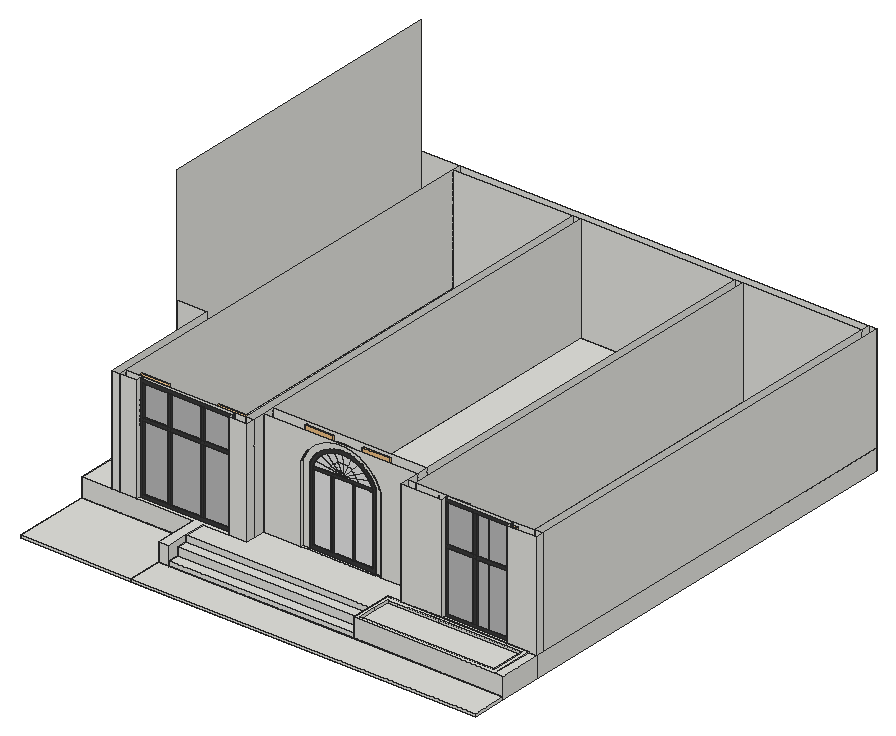
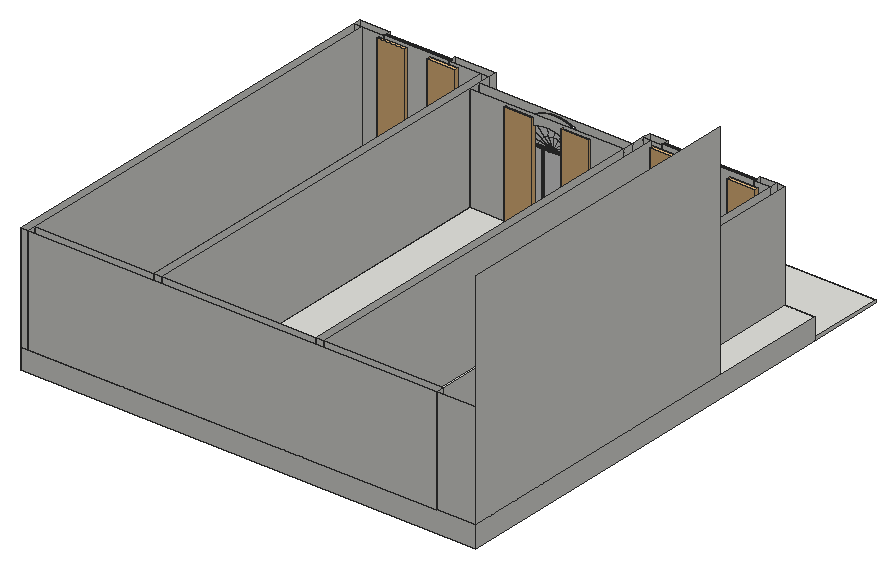
# SketchUp Ruby script. Lengths in inches.
U = 1.inch
M = Sketchup.active_model
def pt(a) = Geom::Point3d.new(a.map { |v| v * U })
def face(e, loops, mat)
  f = e.add_face(loops[0].map { |a| pt(a) })
  loops[1..].each { |l| e.add_face(l.map { |a| pt(a) }).erase! }
  f.material = f.back_material = mat if mat
  f
end
# faces: each face lists its corners as indices into pts; further lists are holes
def faces(e, pts, list, mat = nil) = list.each { |f| face(e, (f[0].is_a?(Array) ? f : [f]).map { |l| l.map { |i| pts[i] } }, mat) }
# xy, xz, yz: faces in a plane at the given z, y or x. An outline is a flat list of corners, or four numbers for a rectangle; further outlines are holes
def ring(l) = l.size == 4 ? [[l[0], l[1]], [l[2], l[1]], [l[2], l[3]], [l[0], l[3]]] : l.each_slice(2).to_a
def flat(e, list, mat, &to3) = list.each { |f| face(e, (f[0].is_a?(Array) ? f : [f]).map { |l| ring(l).map { |u, v| to3.(u, v) } }, mat) }
def xy(e, z, list, mat = nil) = flat(e, list, mat) { |x, y| [x, y, z] }
def xz(e, y, list, mat = nil) = flat(e, list, mat) { |x, z| [x, y, z] }
def yz(e, x, list, mat = nil) = flat(e, list, mat) { |y, z| [x, y, z] }
def lines(e, pts, list) = list.each { |a, b| e.add_line(pt(pts[a]), pt(pts[b])) }
# prism: a flat outline (further loops are holes) pulled along v
def prism(e, loops, v, mat = nil)
  f = face(e, loops, mat); d = Geom::Vector3d.new(v.map { |x| x * U })
  f.pushpull(f.normal.samedirection?(d) ? d.length : -d.length)
end
def box(e, o, s, mat = nil) = prism(e, [[o, [o[0] + s[0], o[1], o[2]], [o[0] + s[0], o[1] + s[1], o[2]], [o[0], o[1] + s[1], o[2]]]], [0, 0, s[2]], mat)
def at(x, y, z, deg = 0) = Geom::Transformation.translation(pt([x, y, z])) * Geom::Transformation.rotation(ORIGIN, Z_AXIS, deg.degrees)
def axes(o, x, y, z) = Geom::Transformation.new([*x, 0, *y, 0, *z, 0, *pt(o).to_a, 1])
def part(name) = M.definitions.add(name)
# library, detail: a bought-in or finely detailed component or shape, given as its bounding box
def library(name, o, s) = part(name).tap { |d| box(d.entities, o, s) }
def detail(e, o, s) = box(e.add_group.entities, o, s)
def put(e, d, t, mat = nil) = e.add_instance(d, t).tap { |i| i.material = mat if mat }
def group(e, t, mat = nil) = e.add_group.tap { |g| g.transformation = t; g.material = mat if mat }.entities
root = M.entities
M.materials.add("[Color M07]").color = [58, 58, 58]
M.materials.add("[Mirror 01]").color = [185, 185, 185]
M.materials.add("[Mirror 02]").color = [229, 229, 229]
c1 = library("Curtains 004",[-15.59,-2.26,0],[31.18,4.52,116.91])
xy(root,-24,[[2.97,0,128.4,86.25],[128.4,0,517.41,38.25],[128.4,38.25,128.4,86.25,2.97,86.25,2.97,566.25,517.41,566.25,517.41,86.25,140.65,86.25,140.65,38.25],[140.65,38.25,348.83,86.25],[348.83,38.25,517.41,86.25]])
xy(root,-20.66,[[2.97,0,128.4,86.25],[128.4,0,517.41,38.25]])
xy(root,-15.28,[[140.65,38.25,348.83,50.25]])
xy(root,-6.56,[[140.65,50.25,348.83,62.25]])
xy(root,-2.4375,[[353.04,42.45,504.2,82.05]])
xy(root,0,[[128.4,38.25,140.65,38.25,140.65,86.25,169.68,86.25,169.68,90.75,65.51,90.75,65.51,86.25,128.4,86.25],[508.41,38.25,517.41,86.25],[140.65,62.25,348.83,62.25,348.83,86.25,364.41,86.25,364.41,109.85,190.41,109.85,190.41,86.25,140.65,86.25],[2.97,86.25,37.41,220.92],[37.41,86.25,37.41,220.92,2.97,220.92,2.97,566.25,46.41,566.25,46.41,86.25],
  [46.41,86.25,65.51,95.25],[169.68,86.25,190.41,95.25],[364.41,86.25,409.78,95.25],[409.78,86.25,483.95,90.75],[483.95,86.25,508.41,95.25],
  [508.41,86.25,517.41,95.25],[46.41,95.25,181.41,557.25],[181.41,95.25,190.41,557.25],[364.41,95.25,373.41,557.25],[373.41,95.25,508.41,557.25],
  [508.41,95.25,517.41,566.25],[232.59,109.85,239.71,112.66],[239.71,109.85,314.84,112.66],[314.84,109.85,321.96,112.66],[239.71,113.47,314.84,122.61],
  [190.41,122.61,364.41,557.25],[46.41,557.25,508.41,566.25]])
xy(root,0,[[65.51,90.75,169.68,94.4375],[409.78,90.75,483.95,94.5625],[239.71,112.66,314.84,113.47]],"[Color M07]")
xy(root,0.875,[[[348.83,38.25,508.41,86.25],[353.04,42.45,504.2,82.05]]])
xy(root,3.13,[[412.91,90.75,441.92,92.125],[446.86,90.75,480.82,92.125]],"[Color M07]")
xy(root,3.65,[[69.16,90.75,96.8,92.5625],[100.57,90.75,134.3,92.5625],[137.83,90.75,166.03,92.5625]],"[Color M07]")
xy(root,3.99,[[263.76,112.66,266.13,113.47],[288.32,112.66,290.13,113.47]])
xy(root,3.99,[[243.71,112.66,263.76,113.47],[266.13,112.66,288.32,113.47],[290.13,112.66,310.84,113.47]],"[Color M07]")
xy(root,70.47,[[412.91,90.75,441.92,92.125],[446.86,90.75,480.82,92.125]],"[Color M07]")
xy(root,74.03,[[412.91,90.75,441.92,92.125],[446.86,90.75,480.82,92.125]],"[Color M07]")
xy(root,78.26,[[69.16,90.75,96.8,92.5625],[100.57,90.75,134.3,92.5625],[137.83,90.75,166.03,92.5625]],"[Color M07]")
xy(root,81.33,[[243.71,112.66,263.76,113.47],[266.13,112.66,288.32,113.47],[290.13,112.66,310.84,113.47]],"[Color M07]")
xy(root,81.69,[[69.16,90.75,96.8,92.5625],[100.57,90.75,134.3,92.5625],[137.83,90.75,166.03,92.5625]],"[Color M07]")
xz(root,0,[[2.97,-24,128.4,-20.66],[128.4,-24,517.41,-20.66]])
xz(root,38.25,[[128.4,-24,140.65,-20.66],[140.65,-24,348.83,-20.66],[348.83,-24,517.41,-20.66],[128.4,-20.66,140.65,0],[140.65,-20.66,348.83,-15.28],
  [348.83,-20.66,517.41,-20.66,517.41,0,508.41,0,508.41,0.875,348.83,0.875]])
xz(root,42.45,[[353.04,-2.4375,504.2,0.875]])
xz(root,50.25,[[140.65,-15.28,348.83,-6.56]])
xz(root,62.25,[[140.65,-6.56,348.83,0]])
xz(root,82.05,[[353.04,-2.4375,364.41,0.875],[364.41,-2.4375,409.78,0.875],[409.78,-2.4375,483.95,0.875],[483.95,-2.4375,504.2,0.875]])
xz(root,86.25,[[2.97,-24,128.4,-20.66],[348.83,-24,517.41,0],[2.97,-20.66,128.4,0],[37.41,0,46.41,120],[46.41,0,65.51,120],
  [169.68,0,190.41,120],[348.83,0,364.41,0.875],[364.41,0,409.78,0.875],[409.78,0,483.95,0.875],[483.95,0,508.41,0.875],
  [508.41,0,517.41,0,517.41,120,483.95,120,483.95,0.875,508.41,0.875],[364.41,0.875,409.78,120]])
xz(root,90.75,[[[65.51,0,169.68,120],[69.16,3.65,166.03,116.35]],[[409.78,0,483.95,120],[412.91,3.13,480.82,116.87]],[441.92,3.13,446.86,70.47],[96.8,3.65,100.57,78.26],[134.3,3.65,137.83,78.26],
  [412.91,70.47,441.92,74.03],[441.92,70.47,446.86,74.03],[446.86,70.47,480.82,74.03],[441.92,74.03,446.86,116.87],[69.16,78.26,96.8,81.69],
  [96.8,78.26,100.57,81.69],[100.57,78.26,134.3,81.69],[134.3,78.26,137.83,81.69],[137.83,78.26,166.03,81.69],[96.8,81.69,100.57,116.35],
  [134.3,81.69,137.83,116.35]],"[Color M07]")
xz(root,92.125,[[412.91,3.13,441.92,70.47],[446.86,3.13,480.82,70.47],[412.91,74.03,441.92,116.87],[446.86,74.03,480.82,116.87]],"[Mirror 01]")
xz(root,92.5625,[[69.16,3.65,96.8,78.26],[100.57,3.65,134.3,78.26],[137.83,3.65,166.03,78.26],[69.16,81.69,96.8,116.35],[100.57,81.69,134.3,116.35],
  [137.83,81.69,166.03,116.35]],"[Mirror 01]")
xz(root,94.4375,[[65.51,0,169.68,120]])
xz(root,94.5625,[[409.78,0,483.95,120]])
xz(root,95.25,[[46.41,0,65.51,120],[169.68,0,181.41,120],[181.41,0,190.41,120],[364.41,0,373.41,120],[373.41,0,409.78,120],
  [483.95,0,508.41,120],[508.41,0,517.41,120]])
xz(root,109.85,[[232.59,-7.12,321.96,0],[190.41,0,232.59,0,232.59,86.36,233.42,88.57,233.86,89.64,234.31,90.69,234.8,91.74,235.31,92.77,235.84,93.79,236.4,94.8,236.98,95.79,237.59,96.77,238.22,97.73,238.88,98.68,239.56,99.61,240.26,100.52,240.98,101.42,241.72,102.3,242.49,103.16,243.27,104,244.08,104.82,244.91,105.62,245.75,106.4,246.62,107.16,247.5,107.9,248.4,108.62,249.32,109.3125,250.25,109.99,251.2,110.64,252.17,111.26,253.15,111.86,254.15,112.44,255.16,112.99,256.18,113.52,257.21,114.03,258.26,114.5,259.32,114.96,260.39,115.38,261.47,115.78,262.56,116.15,263.66,116.5,264.76,116.82,265.88,117.11,267,117.38,268.125,117.62,269.26,117.83,270.39,118.01,271.53,118.16,272.68,118.29,273.83,118.39,274.97,118.46,276.125,118.5,277.28,118.51,278.43,118.5,279.58,118.46,280.73,118.39,281.875,118.29,283.02,118.16,284.16,118.01,285.3,117.83,286.43,117.62,287.55,117.38,288.67,117.11,289.79,116.82,290.89,116.5,291.99,116.15,293.08,115.78,294.16,115.38,295.23,114.96,296.29,114.5,297.34,114.03,298.37,113.52,299.4,112.99,300.41,112.44,301.4,111.86,302.38,111.26,303.35,110.64,304.3,109.99,305.23,109.3125,306.15,108.62,307.05,107.9,307.94,107.16,308.8,106.4,309.65,105.62,310.47,104.82,311.28,104,312.0625,103.16,312.83,102.3,313.57,101.42,314.3,100.52,315,99.61,315.67,98.68,316.33,97.73,316.96,96.77,317.57,95.79,318.15,94.8,318.71,93.79,319.24,92.77,319.75,91.74,320.24,90.69,320.7,89.64,321.13,88.57,321.96,86.36,321.96,0,364.41,0,364.41,120,190.41,120]])
xz(root,112.66,[[232.59,0,239.71,0,239.71,85.0625,240.06,85.98,240.42,86.88,240.8125,87.78,241.22,88.67,241.66,89.54,242.11,90.41,242.58,91.26,243.08,92.1,243.6,92.93,244.13,93.75,244.6875,94.56,245.26,95.35,245.86,96.12,246.47,96.88,247.1,97.63,247.75,98.36,248.42,99.07,249.1,99.77,249.8,100.45,250.52,101.11,251.25,101.76,252,102.38,252.77,102.99,253.55,103.58,254.34,104.15,255.15,104.71,255.97,105.24,256.8,105.75,257.65,106.24,258.5,106.71,259.37,107.16,260.25,107.58,261.14,107.99,262.04,108.37,262.94,108.73,263.86,109.07,264.79,109.39,265.72,109.68,266.66,109.95,267.6,110.2,268.55,110.43,269.51,110.63,270.47,110.81,271.43,110.96,272.4,111.09,273.375,111.2,274.35,111.28,275.32,111.34,276.3,111.38,277.28,111.39,278.25,111.38,279.23,111.34,280.2,111.28,281.18,111.2,282.15,111.09,283.12,110.96,284.08,110.81,285.04,110.63,286,110.43,286.95,110.2,287.9,109.95,288.83,109.68,289.77,109.39,290.69,109.07,291.61,108.73,292.51,108.37,293.41,107.99,294.3,107.58,295.18,107.16,296.05,106.71,296.91,106.24,297.75,105.75,298.58,105.24,299.4,104.71,300.21,104.15,301,103.58,301.78,102.99,302.55,102.38,303.3,101.76,304.03,101.11,304.75,100.45,305.45,99.77,306.13,99.07,306.8,98.36,307.45,97.63,308.08,96.88,308.7,96.12,309.29,95.35,309.87,94.56,310.42,93.75,310.96,92.93,311.47,92.1,311.97,91.26,312.44,90.41,312.9,89.54,313.33,88.67,313.74,87.78,314.13,86.88,314.49,85.98,314.84,85.0625,314.84,0,321.96,0,321.96,86.36,321.13,88.57,320.7,89.64,320.24,90.69,319.75,91.74,319.24,92.77,318.71,93.79,318.15,94.8,317.57,95.79,316.96,96.77,316.33,97.73,315.67,98.68,315,99.61,314.3,100.52,313.57,101.42,312.83,102.3,312.0625,103.16,311.28,104,310.47,104.82,309.65,105.62,308.8,106.4,307.94,107.16,307.05,107.9,306.15,108.62,305.23,109.3125,304.3,109.99,303.35,110.64,302.38,111.26,301.4,111.86,300.41,112.44,299.4,112.99,298.37,113.52,297.34,114.03,296.29,114.5,295.23,114.96,294.16,115.38,293.08,115.78,291.99,116.15,290.89,116.5,289.79,116.82,288.67,117.11,287.55,117.38,286.43,117.62,285.3,117.83,284.16,118.01,283.02,118.16,281.875,118.29,280.73,118.39,279.58,118.46,278.43,118.5,277.28,118.51,276.125,118.5,274.97,118.46,273.83,118.39,272.68,118.29,271.53,118.16,270.39,118.01,269.26,117.83,268.125,117.62,267,117.38,265.88,117.11,264.76,116.82,263.66,116.5,262.56,116.15,261.47,115.78,260.39,115.38,259.32,114.96,258.26,114.5,257.21,114.03,256.18,113.52,255.16,112.99,254.15,112.44,253.15,111.86,252.17,111.26,251.2,110.64,250.25,109.99,249.32,109.3125,248.4,108.62,247.5,107.9,246.62,107.16,245.75,106.4,244.91,105.62,244.08,104.82,243.27,104,242.49,103.16,241.72,102.3,240.98,101.42,240.26,100.52,239.56,99.61,238.88,98.68,238.22,97.73,237.59,96.77,236.98,95.79,236.4,94.8,235.84,93.79,235.31,92.77,234.8,91.74,234.31,90.69,233.86,89.64,233.42,88.57,232.59,86.36]])
xz(root,112.66,[[[239.71,0,314.84,0,314.84,85.0625,314.49,85.98,314.13,86.88,313.74,87.78,313.33,88.67,312.9,89.54,312.44,90.41,311.97,91.26,311.47,92.1,310.96,92.93,310.42,93.75,309.87,94.56,309.29,95.35,308.7,96.12,308.08,96.88,307.45,97.63,306.8,98.36,306.13,99.07,305.45,99.77,304.75,100.45,304.03,101.11,303.3,101.76,302.55,102.38,301.78,102.99,301,103.58,300.21,104.15,299.4,104.71,298.58,105.24,297.75,105.75,296.91,106.24,296.05,106.71,295.18,107.16,294.3,107.58,293.41,107.99,292.51,108.37,291.61,108.73,290.69,109.07,289.77,109.39,288.83,109.68,287.9,109.95,286.95,110.2,286,110.43,285.04,110.63,284.08,110.81,283.12,110.96,282.15,111.09,281.18,111.2,280.2,111.28,279.23,111.34,278.25,111.38,277.28,111.39,276.3,111.38,275.32,111.34,274.35,111.28,273.375,111.2,272.4,111.09,271.43,110.96,270.47,110.81,269.51,110.63,268.55,110.43,267.6,110.2,266.66,109.95,265.72,109.68,264.79,109.39,263.86,109.07,262.94,108.73,262.04,108.37,261.14,107.99,260.25,107.58,259.37,107.16,258.5,106.71,257.65,106.24,256.8,105.75,255.97,105.24,255.15,104.71,254.34,104.15,253.55,103.58,252.77,102.99,252,102.38,251.25,101.76,250.52,101.11,249.8,100.45,249.1,99.77,248.42,99.07,247.75,98.36,247.1,97.63,246.47,96.88,245.86,96.12,245.26,95.35,244.6875,94.56,244.13,93.75,243.6,92.93,243.08,92.1,242.58,91.26,242.11,90.41,241.66,89.54,241.22,88.67,240.8125,87.78,240.42,86.88,240.06,85.98,239.71,85.0625],[243.71,3.99,243.71,84.33,243.78,84.52,244.11,85.34,244.46,86.14,244.83,86.94,245.22,87.73,245.625,88.51,246.05,89.28,246.5,90.04,246.96,90.78,247.44,91.52,247.94,92.24,248.46,92.95,249,93.65,249.55,94.34,250.12,95.01,250.7,95.67,251.3,96.31,251.92,96.9375,252.55,97.55,253.2,98.15,253.86,98.73,254.53,99.29,255.22,99.84,255.92,100.37,256.63,100.88,257.36,101.38,258.1,101.86,258.85,102.32,259.61,102.76,260.38,103.18,261.16,103.58,261.95,103.97,262.75,104.33,263.5625,104.68,264.38,105,265.2,105.31,266.03,105.59,266.875,105.86,267.72,106.1,268.57,106.33,269.42,106.53,270.28,106.71,271.15,106.87,272.02,107.01,272.89,107.13,273.76,107.22,274.64,107.3,275.52,107.35,276.4,107.39,277.28,107.4,278.16,107.39,279.03,107.35,279.91,107.3,280.79,107.22,281.66,107.13,282.53,107.01,283.4,106.87,284.27,106.71,285.13,106.53,285.98,106.33,286.83,106.1,287.68,105.86,288.52,105.59,289.35,105.31,290.17,105,290.99,104.68,291.8,104.33,292.6,103.97,293.39,103.58,294.17,103.18,294.94,102.76,295.7,102.32,296.45,101.86,297.19,101.38,297.92,100.88,298.63,100.37,299.33,99.84,300.02,99.29,300.7,98.73,301.36,98.15,302,97.55,302.63,96.9375,303.25,96.31,303.85,95.67,304.43,95.01,305,94.34,305.55,93.65,306.09,92.95,306.61,92.24,307.11,91.52,307.59,90.78,308.05,90.04,308.5,89.28,308.93,88.51,309.33,87.73,309.72,86.94,310.09,86.14,310.44,85.34,310.77,84.52,310.84,84.33,310.84,3.99]],[263.76,3.99,266.13,81.33],[288.32,3.99,290.13,81.33],[243.71,81.33,310.84,81.33,310.84,84.33,310.77,84.52,294.01,84.48,260.47,84.38,243.71,84.33]],"[Color M07]")
xz(root,113.47,[[[239.71,0,239.71,85.0625,240.06,85.98,240.42,86.88,240.8125,87.78,241.22,88.67,241.66,89.54,242.11,90.41,242.58,91.26,243.08,92.1,243.6,92.93,244.13,93.75,244.6875,94.56,245.26,95.35,245.86,96.12,246.47,96.88,247.1,97.63,247.75,98.36,248.42,99.07,249.1,99.77,249.8,100.45,250.52,101.11,251.25,101.76,252,102.38,252.77,102.99,253.55,103.58,254.34,104.15,255.15,104.71,255.97,105.24,256.8,105.75,257.65,106.24,258.5,106.71,259.37,107.16,260.25,107.58,261.14,107.99,262.04,108.37,262.94,108.73,263.86,109.07,264.79,109.39,265.72,109.68,266.66,109.95,267.6,110.2,268.55,110.43,269.51,110.63,270.47,110.81,271.43,110.96,272.4,111.09,273.375,111.2,274.35,111.28,275.32,111.34,276.3,111.38,277.28,111.39,278.25,111.38,279.23,111.34,280.2,111.28,281.18,111.2,282.15,111.09,283.12,110.96,284.08,110.81,285.04,110.63,286,110.43,286.95,110.2,287.9,109.95,288.83,109.68,289.77,109.39,290.69,109.07,291.61,108.73,292.51,108.37,293.41,107.99,294.3,107.58,295.18,107.16,296.05,106.71,296.91,106.24,297.75,105.75,298.58,105.24,299.4,104.71,300.21,104.15,301,103.58,301.78,102.99,302.55,102.38,303.3,101.76,304.03,101.11,304.75,100.45,305.45,99.77,306.13,99.07,306.8,98.36,307.45,97.63,308.08,96.88,308.7,96.12,309.29,95.35,309.87,94.56,310.42,93.75,310.96,92.93,311.47,92.1,311.97,91.26,312.44,90.41,312.9,89.54,313.33,88.67,313.74,87.78,314.13,86.88,314.49,85.98,314.84,85.0625,314.84,0],[243.71,3.99,310.84,3.99,310.84,84.33,310.77,84.52,310.44,85.34,310.09,86.14,309.72,86.94,309.33,87.73,308.93,88.51,308.5,89.28,308.05,90.04,307.59,90.78,307.11,91.52,306.61,92.24,306.09,92.95,305.55,93.65,305,94.34,304.43,95.01,303.85,95.67,303.25,96.31,302.63,96.9375,302,97.55,301.36,98.15,300.7,98.73,300.02,99.29,299.33,99.84,298.63,100.37,297.92,100.88,297.19,101.38,296.45,101.86,295.7,102.32,294.94,102.76,294.17,103.18,293.39,103.58,292.6,103.97,291.8,104.33,290.99,104.68,290.17,105,289.35,105.31,288.52,105.59,287.68,105.86,286.83,106.1,285.98,106.33,285.13,106.53,284.27,106.71,283.4,106.87,282.53,107.01,281.66,107.13,280.79,107.22,279.91,107.3,279.03,107.35,278.16,107.39,277.28,107.4,276.4,107.39,275.52,107.35,274.64,107.3,273.76,107.22,272.89,107.13,272.02,107.01,271.15,106.87,270.28,106.71,269.42,106.53,268.57,106.33,267.72,106.1,266.875,105.86,266.03,105.59,265.2,105.31,264.38,105,263.5625,104.68,262.75,104.33,261.95,103.97,261.16,103.58,260.38,103.18,259.61,102.76,258.85,102.32,258.1,101.86,257.36,101.38,256.63,100.88,255.92,100.37,255.22,99.84,254.53,99.29,253.86,98.73,253.2,98.15,252.55,97.55,251.92,96.9375,251.3,96.31,250.7,95.67,250.12,95.01,249.55,94.34,249,93.65,248.46,92.95,247.94,92.24,247.44,91.52,246.96,90.78,246.5,90.04,246.05,89.28,245.625,88.51,245.22,87.73,244.83,86.94,244.46,86.14,244.11,85.34,243.78,84.52,243.71,84.33]]])
xz(root,113.47,[[243.71,3.99,263.76,81.33],[266.13,3.99,288.32,81.33],[290.13,3.99,310.84,81.33],[243.71,84.33,260.47,84.38,261.55,87.29,246.5,90.04,246.05,89.28,245.625,88.51,245.22,87.73,244.83,86.94,244.46,86.14,244.11,85.34,243.78,84.52],[260.47,84.38,277.24,84.43,261.55,87.29],
  [277.24,84.43,263.5625,90.69,261.79,87.96,261.55,87.29],[277.24,84.43,266.78,93.95,266.58,93.82,263.86,91.16,263.5625,90.69],[277.24,84.43,270.99,96.24,269.82,95.83,266.78,93.95],[277.24,84.43,276.27,97.41,273.42,97.08,270.99,96.24],[277.24,84.43,282.14,96.71,280.99,97.1,277.2,97.51,276.27,97.41],
  [277.24,84.43,286.92,94.45,284.6,95.875,282.14,96.71],[277.24,84.43,290.4,91.4,287.85,93.88,286.92,94.45],[277.24,84.43,292.64,88.09,290.58,91.23,290.4,91.4],[277.24,84.43,294.01,84.48,292.67,88.04,292.64,88.09],[294.01,84.48,310.77,84.52,310.44,85.34,310.09,86.14,309.72,86.94,309.33,87.73,308.93,88.51,308.5,89.28,308.05,90.04,307.59,90.78,307.11,91.52,292.64,88.09,292.67,88.04],
  [261.55,87.29,261.79,87.96,263.5625,90.69,251.3,96.31,250.7,95.67,250.12,95.01,249.55,94.34,249,93.65,248.46,92.95,247.94,92.24,247.44,91.52,246.96,90.78,246.5,90.04],[292.64,88.09,307.11,91.52,306.61,92.24,306.09,92.95,305.55,93.65,305,94.34,304.43,95.01,303.85,95.67,303.25,96.31,302.63,96.9375,302,97.55,290.4,91.4,290.58,91.23],[263.5625,90.69,263.86,91.16,266.58,93.82,266.78,93.95,258.1,101.86,257.36,101.38,256.63,100.88,255.92,100.37,255.22,99.84,254.53,99.29,253.86,98.73,253.2,98.15,252.55,97.55,251.92,96.9375,251.3,96.31],[290.4,91.4,302,97.55,301.36,98.15,300.7,98.73,300.02,99.29,299.33,99.84,298.63,100.37,297.92,100.88,297.19,101.38,296.45,101.86,295.7,102.32,294.94,102.76,286.92,94.45,287.85,93.88],[266.78,93.95,269.82,95.83,270.99,96.24,266.03,105.59,265.2,105.31,264.38,105,263.5625,104.68,262.75,104.33,261.95,103.97,261.16,103.58,260.38,103.18,259.61,102.76,258.85,102.32,258.1,101.86],
  [286.92,94.45,294.94,102.76,294.17,103.18,293.39,103.58,292.6,103.97,291.8,104.33,290.99,104.68,290.17,105,289.35,105.31,288.52,105.59,287.68,105.86,286.83,106.1,285.98,106.33,282.14,96.71,284.6,95.875],[270.99,96.24,273.42,97.08,276.27,97.41,275.52,107.35,274.64,107.3,273.76,107.22,272.89,107.13,272.02,107.01,271.15,106.87,270.28,106.71,269.42,106.53,268.57,106.33,267.72,106.1,266.875,105.86,266.03,105.59],[282.14,96.71,285.98,106.33,285.13,106.53,284.27,106.71,283.4,106.87,282.53,107.01,281.66,107.13,280.79,107.22,279.91,107.3,279.03,107.35,278.16,107.39,277.28,107.4,276.4,107.39,275.52,107.35,276.27,97.41,277.2,97.51,280.99,97.1]],"[Mirror 02]")
xz(root,122.61,[[190.41,0,190.41,120,364.41,120,364.41,0,314.84,0,314.84,85.0625,314.49,85.98,314.13,86.88,313.74,87.78,313.33,88.67,312.9,89.54,312.44,90.41,311.97,91.26,311.47,92.1,310.96,92.93,310.42,93.75,309.87,94.56,309.29,95.35,308.7,96.12,308.08,96.88,307.45,97.63,306.8,98.36,306.13,99.07,305.45,99.77,304.75,100.45,304.03,101.11,303.3,101.76,302.55,102.38,301.78,102.99,301,103.58,300.21,104.15,299.4,104.71,298.58,105.24,297.75,105.75,296.91,106.24,296.05,106.71,295.18,107.16,294.3,107.58,293.41,107.99,292.51,108.37,291.61,108.73,290.69,109.07,289.77,109.39,288.83,109.68,287.9,109.95,286.95,110.2,286,110.43,285.04,110.63,284.08,110.81,283.12,110.96,282.15,111.09,281.18,111.2,280.2,111.28,279.23,111.34,278.25,111.38,277.28,111.39,276.3,111.38,275.32,111.34,274.35,111.28,273.375,111.2,272.4,111.09,271.43,110.96,270.47,110.81,269.51,110.63,268.55,110.43,267.6,110.2,266.66,109.95,265.72,109.68,264.79,109.39,263.86,109.07,262.94,108.73,262.04,108.37,261.14,107.99,260.25,107.58,259.37,107.16,258.5,106.71,257.65,106.24,256.8,105.75,255.97,105.24,255.15,104.71,254.34,104.15,253.55,103.58,252.77,102.99,252,102.38,251.25,101.76,250.52,101.11,249.8,100.45,249.1,99.77,248.42,99.07,247.75,98.36,247.1,97.63,246.47,96.88,245.86,96.12,245.26,95.35,244.6875,94.56,244.13,93.75,243.6,92.93,243.08,92.1,242.58,91.26,242.11,90.41,241.66,89.54,241.22,88.67,240.8125,87.78,240.42,86.88,240.06,85.98,239.71,85.0625,239.71,0]])
xz(root,220.92,[[2.97,0,37.41,120]])
xz(root,557.25,[[46.41,0,181.41,120],[181.41,0,190.41,120],[190.41,0,364.41,120],[364.41,0,373.41,120],[373.41,0,508.41,120]])
xz(root,566.25,[[2.97,-24,517.41,0],[2.97,0,46.41,120],[46.41,0,508.41,120],[508.41,0,517.41,120]])
yz(root,2.97,[[0,-24,86.25,-20.66],[86.25,-24,566.25,0],[220.92,0,566.25,252]])
yz(root,37.41,[[86.25,0,220.92,120]])
yz(root,46.41,[[86.25,0,95.25,120],[95.25,0,557.25,120],[557.25,0,566.25,120]])
yz(root,65.51,[[86.25,0,90.75,120],[94.4375,0,95.25,120]])
yz(root,65.51,[[90.75,0,94.4375,120]],"[Color M07]")
yz(root,69.16,[[90.75,3.65,92.5625,78.26],[90.75,81.69,92.5625,116.35]],"[Color M07]")
yz(root,96.8,[[90.75,3.65,92.5625,78.26],[90.75,81.69,92.5625,116.35]],"[Color M07]")
yz(root,100.57,[[90.75,3.65,92.5625,78.26],[90.75,81.69,92.5625,116.35]],"[Color M07]")
yz(root,128.4,[[0,-24,38.25,-20.66],[38.25,-24,86.25,-20.66],[38.25,-20.66,86.25,0]])
yz(root,134.3,[[90.75,3.65,92.5625,78.26],[90.75,81.69,92.5625,116.35]],"[Color M07]")
yz(root,137.83,[[90.75,3.65,92.5625,78.26],[90.75,81.69,92.5625,116.35]],"[Color M07]")
yz(root,140.65,[[38.25,-24,86.25,-24,86.25,0,62.25,0,62.25,-6.56,50.25,-6.56,50.25,-15.28,38.25,-15.28],[38.25,-15.28,50.25,-15.28,50.25,-6.56,62.25,-6.56,62.25,0,38.25,0]])
yz(root,166.03,[[90.75,3.65,92.5625,78.26],[90.75,81.69,92.5625,116.35]],"[Color M07]")
yz(root,169.68,[[86.25,0,90.75,120],[94.4375,0,95.25,120]])
yz(root,169.68,[[90.75,0,94.4375,120]],"[Color M07]")
yz(root,181.41,[[95.25,0,557.25,120]])
yz(root,190.41,[[86.25,0,95.25,120],[95.25,0,109.85,120],[109.85,0,122.61,120],[122.61,0,557.25,120]])
yz(root,232.59,[[109.85,0,112.66,86.36]])
yz(root,239.71,[[113.47,0,122.61,85.0625]])
yz(root,239.71,[[112.66,0,113.47,85.0625]],"[Color M07]")
yz(root,243.71,[[112.66,81.33,113.47,84.33]])
yz(root,243.71,[[112.66,3.99,113.47,81.33]],"[Color M07]")
yz(root,263.76,[[112.66,3.99,113.47,81.33]],"[Color M07]")
yz(root,266.13,[[112.66,3.99,113.47,81.33]],"[Color M07]")
yz(root,288.32,[[112.66,3.99,113.47,81.33]],"[Color M07]")
yz(root,290.13,[[112.66,3.99,113.47,81.33]],"[Color M07]")
yz(root,310.84,[[112.66,81.33,113.47,84.33]])
yz(root,310.84,[[112.66,3.99,113.47,81.33]],"[Color M07]")
yz(root,314.84,[[113.47,0,122.61,85.0625]])
yz(root,314.84,[[112.66,0,113.47,85.0625]],"[Color M07]")
yz(root,321.96,[[109.85,0,112.66,86.36]])
yz(root,348.83,[[38.25,-24,86.25,-24,86.25,0,62.25,0,62.25,-6.56,50.25,-6.56,50.25,-15.28,38.25,-15.28],[38.25,-15.28,50.25,-6.56],[38.25,-6.56,62.25,0.875],[62.25,0,86.25,0.875]])
yz(root,353.04,[[42.45,-2.4375,62.25,0.875],[62.25,-2.4375,82.05,0.875]])
yz(root,364.41,[[86.25,0,95.25,120],[95.25,0,109.85,120],[109.85,0,122.61,120],[122.61,0,557.25,120]])
yz(root,373.41,[[95.25,0,557.25,120]])
yz(root,409.78,[[86.25,0,90.75,120],[94.5625,0,95.25,120]])
yz(root,409.78,[[90.75,0,94.5625,120]],"[Color M07]")
yz(root,412.91,[[90.75,3.13,92.125,70.47],[90.75,74.03,92.125,116.87]],"[Color M07]")
yz(root,441.92,[[90.75,3.13,92.125,70.47],[90.75,74.03,92.125,116.87]],"[Color M07]")
yz(root,446.86,[[90.75,3.13,92.125,70.47],[90.75,74.03,92.125,116.87]],"[Color M07]")
yz(root,480.82,[[90.75,3.13,92.125,70.47],[90.75,74.03,92.125,116.87]],"[Color M07]")
yz(root,483.95,[[86.25,0,90.75,120],[94.5625,0,95.25,120]])
yz(root,483.95,[[90.75,0,94.5625,120]],"[Color M07]")
yz(root,504.2,[[42.45,-2.4375,82.05,0.875]])
yz(root,508.41,[[38.25,0,86.25,0.875],[95.25,0,557.25,120],[557.25,0,566.25,120]])
yz(root,517.41,[[0,-24,38.25,-20.66],[38.25,-24,86.25,0],[86.25,-24,566.25,0],[86.25,0,95.25,120],[95.25,0,566.25,120]])
p = [[243.71,113.47,84.33],[243.78,113.47,84.52],[243.78,112.66,84.52],[243.71,112.66,84.33],[260.47,113.47,84.38],[260.47,112.66,84.38],
  [310.77,113.47,84.52],[310.84,113.47,84.33],[310.84,112.66,84.33],[310.77,112.66,84.52],[277.24,113.47,84.43],[277.24,112.66,84.43],
  [294.01,113.47,84.48],[294.01,112.66,84.48],[244.11,113.47,85.34],[244.11,112.66,85.34],[310.44,113.47,85.34],[310.44,112.66,85.34],
  [239.71,113.47,85.0625],[240.06,113.47,85.98],[240.06,112.66,85.98],[239.71,112.66,85.0625],[314.49,113.47,85.98],[314.84,113.47,85.0625],
  [314.84,112.66,85.0625],[314.49,112.66,85.98],[240.06,122.61,85.98],[239.71,122.61,85.0625],[314.84,122.61,85.0625],[314.49,122.61,85.98],
  [244.46,113.47,86.14],[244.46,112.66,86.14],[310.09,113.47,86.14],[310.09,112.66,86.14],[240.42,113.47,86.88],[240.42,112.66,86.88],
  [314.13,113.47,86.88],[314.13,112.66,86.88],[240.42,122.61,86.88],[314.13,122.61,86.88],[244.83,113.47,86.94],[244.83,112.66,86.94],
  [309.72,113.47,86.94],[309.72,112.66,86.94],[233.42,109.85,88.57],[232.59,109.85,86.36],[232.59,112.66,86.36],[233.42,112.66,88.57],
  [321.96,109.85,86.36],[321.13,109.85,88.57],[321.13,112.66,88.57],[321.96,112.66,86.36],[240.8125,113.47,87.78],[240.8125,112.66,87.78],
  [245.22,113.47,87.73],[245.22,112.66,87.73],[309.33,113.47,87.73],[309.33,112.66,87.73],[313.74,113.47,87.78],[313.74,112.66,87.78],
  [240.8125,122.61,87.78],[313.74,122.61,87.78],[245.625,113.47,88.51],[245.625,112.66,88.51],[308.93,113.47,88.51],[308.93,112.66,88.51],
  [241.22,113.47,88.67],[241.22,112.66,88.67],[313.33,113.47,88.67],[313.33,112.66,88.67],[241.22,122.61,88.67],[313.33,122.61,88.67],
  [246.05,113.47,89.28],[246.05,112.66,89.28],[308.5,113.47,89.28],[308.5,112.66,89.28],[233.86,109.85,89.64],[233.86,112.66,89.64],
  [320.7,109.85,89.64],[320.7,112.66,89.64],[241.66,113.47,89.54],[241.66,112.66,89.54],[312.9,113.47,89.54],[312.9,112.66,89.54],
  [241.66,122.61,89.54],[312.9,122.61,89.54],[246.5,113.47,90.04],[246.5,112.66,90.04],[308.05,113.47,90.04],[308.05,112.66,90.04],
  [242.11,113.47,90.41],[242.11,112.66,90.41],[312.44,113.47,90.41],[312.44,112.66,90.41],[242.11,122.61,90.41],[312.44,122.61,90.41],
  [234.31,109.85,90.69],[234.31,112.66,90.69],[320.24,109.85,90.69],[320.24,112.66,90.69],[246.96,113.47,90.78],[246.96,112.66,90.78],
  [307.59,113.47,90.78],[307.59,112.66,90.78],[242.58,113.47,91.26],[242.58,112.66,91.26],[311.97,113.47,91.26],[311.97,112.66,91.26],
  [242.58,122.61,91.26],[311.97,122.61,91.26],[234.8,109.85,91.74],[234.8,112.66,91.74],[319.75,109.85,91.74],[319.75,112.66,91.74],
  [247.44,113.47,91.52],[247.44,112.66,91.52],[307.11,113.47,91.52],[307.11,112.66,91.52],[243.08,113.47,92.1],[243.08,112.66,92.1],
  [311.47,113.47,92.1],[311.47,112.66,92.1],[243.08,122.61,92.1],[311.47,122.61,92.1],[247.94,113.47,92.24],[247.94,112.66,92.24],
  [306.61,113.47,92.24],[306.61,112.66,92.24],[235.31,109.85,92.77],[235.31,112.66,92.77],[319.24,109.85,92.77],[319.24,112.66,92.77],
  [243.6,113.47,92.93],[243.6,112.66,92.93],[310.96,113.47,92.93],[310.96,112.66,92.93],[243.6,122.61,92.93],[310.96,122.61,92.93],
  [248.46,113.47,92.95],[248.46,112.66,92.95],[306.09,113.47,92.95],[306.09,112.66,92.95],[235.84,109.85,93.79],[235.84,112.66,93.79],
  [318.71,109.85,93.79],[318.71,112.66,93.79],[244.13,113.47,93.75],[244.13,112.66,93.75],[310.42,113.47,93.75],[310.42,112.66,93.75],
  [244.13,122.61,93.75],[310.42,122.61,93.75],[249,113.47,93.65],[249,112.66,93.65],[305.55,113.47,93.65],[305.55,112.66,93.65],
  [249.55,113.47,94.34],[249.55,112.66,94.34],[305,113.47,94.34],[305,112.66,94.34],[236.4,109.85,94.8],[236.4,112.66,94.8],
  [318.15,109.85,94.8],[318.15,112.66,94.8],[244.6875,113.47,94.56],[244.6875,112.66,94.56],[309.87,113.47,94.56],[309.87,112.66,94.56],
  [244.6875,122.61,94.56],[309.87,122.61,94.56],[250.12,113.47,95.01],[250.12,112.66,95.01],[304.43,113.47,95.01],[304.43,112.66,95.01],
  [245.26,113.47,95.35],[245.26,112.66,95.35],[309.29,113.47,95.35],[309.29,112.66,95.35],[245.26,122.61,95.35],[309.29,122.61,95.35],
  [236.98,109.85,95.79],[236.98,112.66,95.79],[317.57,109.85,95.79],[317.57,112.66,95.79],[250.7,113.47,95.67],[250.7,112.66,95.67],
  [303.85,113.47,95.67],[303.85,112.66,95.67],[245.86,113.47,96.12],[245.86,112.66,96.12],[308.7,113.47,96.12],[308.7,112.66,96.12],
  [245.86,122.61,96.12],[308.7,122.61,96.12],[251.3,113.47,96.31],[251.3,112.66,96.31],[303.25,113.47,96.31],[303.25,112.66,96.31],
  [237.59,109.85,96.77],[237.59,112.66,96.77],[316.96,109.85,96.77],[316.96,112.66,96.77],[246.47,113.47,96.88],[246.47,112.66,96.88],
  [308.08,113.47,96.88],[308.08,112.66,96.88],[246.47,122.61,96.88],[308.08,122.61,96.88],[251.92,113.47,96.9375],[251.92,112.66,96.9375],
  [302.63,113.47,96.9375],[302.63,112.66,96.9375],[238.22,109.85,97.73],[238.22,112.66,97.73],[316.33,109.85,97.73],[316.33,112.66,97.73],
  [247.1,113.47,97.63],[247.1,112.66,97.63],[252.55,113.47,97.55],[252.55,112.66,97.55],[302,113.47,97.55],[302,112.66,97.55],
  [307.45,113.47,97.63],[307.45,112.66,97.63],[247.1,122.61,97.63],[307.45,122.61,97.63],[253.2,113.47,98.15],[253.2,112.66,98.15],
  [301.36,113.47,98.15],[301.36,112.66,98.15],[247.75,113.47,98.36],[247.75,112.66,98.36],[306.8,113.47,98.36],[306.8,112.66,98.36],
  [247.75,122.61,98.36],[306.8,122.61,98.36],[238.88,109.85,98.68],[238.88,112.66,98.68],[315.67,109.85,98.68],[315.67,112.66,98.68],
  [253.86,113.47,98.73],[253.86,112.66,98.73],[300.7,113.47,98.73],[300.7,112.66,98.73],[248.42,113.47,99.07],[248.42,112.66,99.07],
  [306.13,113.47,99.07],[306.13,112.66,99.07],[248.42,122.61,99.07],[306.13,122.61,99.07],[239.56,109.85,99.61],[239.56,112.66,99.61],
  [315,109.85,99.61],[315,112.66,99.61],[254.53,113.47,99.29],[254.53,112.66,99.29],[300.02,113.47,99.29],[300.02,112.66,99.29],
  [249.1,113.47,99.77],[249.1,112.66,99.77],[305.45,113.47,99.77],[305.45,112.66,99.77],[249.1,122.61,99.77],[305.45,122.61,99.77],
  [255.22,113.47,99.84],[255.22,112.66,99.84],[299.33,113.47,99.84],[299.33,112.66,99.84],[240.26,109.85,100.52],[240.26,112.66,100.52],
  [314.3,109.85,100.52],[314.3,112.66,100.52],[249.8,113.47,100.45],[249.8,112.66,100.45],[255.92,113.47,100.37],[255.92,112.66,100.37],
  [298.63,113.47,100.37],[298.63,112.66,100.37],[304.75,113.47,100.45],[304.75,112.66,100.45],[249.8,122.61,100.45],[304.75,122.61,100.45]]
faces(root,p,[[0,1,2,3],[4,0,3,5],[10,4,5,11],[12,10,11,13],[1,14,15,2],[6,12,13,9],[16,6,9,17],[18,19,20,21],
  [22,23,24,25],[14,30,31,15],[32,16,17,33],[19,34,35,20],[36,22,25,37],[30,40,41,31],[42,32,33,43],[34,52,53,35],
  [40,54,55,41],[56,42,43,57],[58,36,37,59],[54,62,63,55],[64,56,57,65],[52,66,67,53],[68,58,59,69],[62,72,73,63],
  [74,64,65,75],[66,80,81,67],[82,68,69,83],[72,86,87,73],[88,74,75,89],[80,90,91,81],[92,82,83,93],[86,100,101,87],
  [102,88,89,103],[90,104,105,91],[106,92,93,107],[100,114,115,101],[116,102,103,117],[104,118,119,105],[120,106,107,121],[114,124,125,115],
  [126,116,117,127],[118,132,133,119],[134,120,121,135],[124,138,139,125],[140,126,127,141],[132,146,147,133],[148,134,135,149],[138,152,153,139],
  [154,140,141,155],[152,156,157,153],[158,154,155,159],[146,164,165,147],[166,148,149,167],[156,170,171,157],[172,158,159,173],[164,174,175,165],
  [176,166,167,177],[170,184,185,171],[186,172,173,187],[174,188,189,175],[190,176,177,191],[184,194,195,185],[196,186,187,197],[188,202,203,189],
  [204,190,191,205],[194,208,209,195],[210,196,197,211],[202,216,217,203],[208,218,219,209],[220,210,211,221],[222,204,205,223],[218,226,227,219],
  [228,220,221,229],[216,230,231,217],[232,222,223,233],[226,240,241,227],[242,228,229,243],[230,244,245,231],[246,232,233,247],[240,254,255,241],
  [256,242,243,257],[244,258,259,245],[260,246,247,261],[254,264,265,255],[266,256,257,267],[258,272,273,259],[264,274,275,265],[276,266,267,277],
  [278,260,261,279]],"[Color M07]")
faces(root,p,[[6,7,8,9],[26,19,18,27],[28,23,22,29],[38,34,19,26],[29,22,36,39],[44,45,46,47],[48,49,50,51],[60,52,34,38],
  [39,36,58,61],[70,66,52,60],[61,58,68,71],[76,44,47,77],[49,78,79,50],[84,80,66,70],[71,68,82,85],[94,90,80,84],
  [85,82,92,95],[96,76,77,97],[78,98,99,79],[108,104,90,94],[95,92,106,109],[110,96,97,111],[98,112,113,99],[122,118,104,108],
  [109,106,120,123],[128,110,111,129],[112,130,131,113],[136,132,118,122],[123,120,134,137],[142,128,129,143],[130,144,145,131],[150,146,132,136],
  [137,134,148,151],[160,142,143,161],[144,162,163,145],[168,164,146,150],[151,148,166,169],[178,174,164,168],[169,166,176,179],[180,160,161,181],
  [162,182,183,163],[192,188,174,178],[179,176,190,193],[198,180,181,199],[182,200,201,183],[206,202,188,192],[193,190,204,207],[212,198,199,213],
  [200,214,215,201],[224,216,202,206],[207,204,222,225],[234,230,216,224],[225,222,232,235],[236,212,213,237],[214,238,239,215],[248,244,230,234],
  [235,232,246,249],[250,236,237,251],[238,252,253,239],[262,258,244,248],[249,246,260,263],[268,250,251,269],[252,270,271,253],[280,272,258,262],
  [263,260,278,281]])
put(root,c1,at(308.52,122.61,0))
put(root,c1,at(243.92,122.61,0))
put(root,c1,at(161.52,100.02,0))
put(root,c1,at(473.85,95.25,0))
put(root,c1,at(415.37,97.62,0))
put(root,c1,at(73.41,101.21,0))
